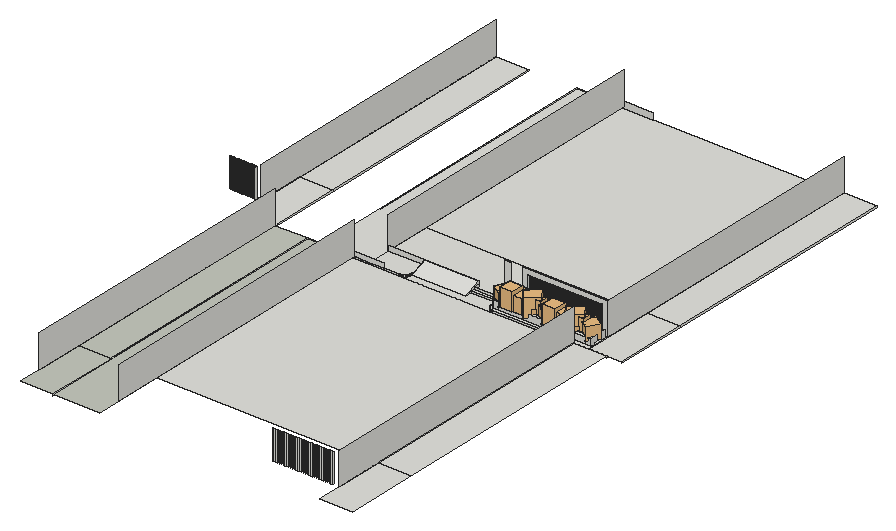
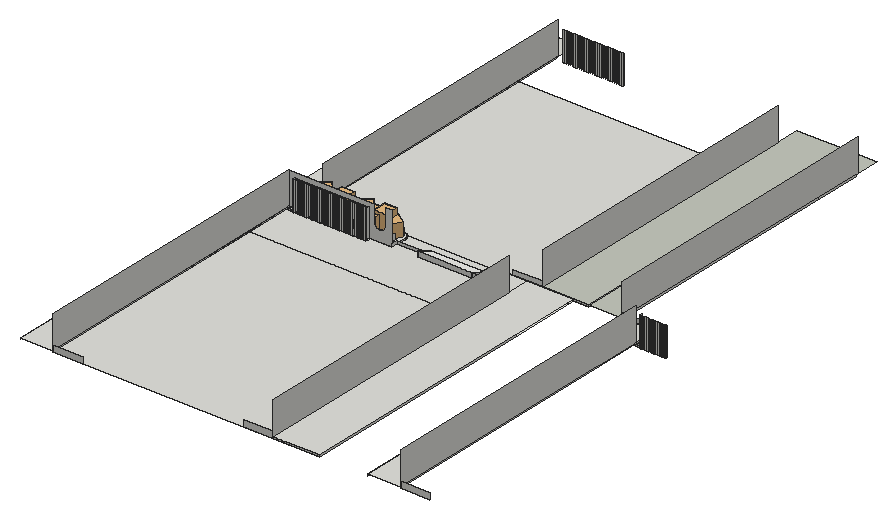
# SketchUp Ruby script. Lengths in inches.
U = 1.inch
M = Sketchup.active_model
def pt(a) = Geom::Point3d.new(a.map { |v| v * U })
def face(e, loops, mat)
  f = e.add_face(loops[0].map { |a| pt(a) })
  loops[1..].each { |l| e.add_face(l.map { |a| pt(a) }).erase! }
  f.material = f.back_material = mat if mat
  f
end
# faces: each face lists its corners as indices into pts; further lists are holes
def faces(e, pts, list, mat = nil) = list.each { |f| face(e, (f[0].is_a?(Array) ? f : [f]).map { |l| l.map { |i| pts[i] } }, mat) }
# xy, xz, yz: faces in a plane at the given z, y or x. An outline is a flat list of corners, or four numbers for a rectangle; further outlines are holes
def ring(l) = l.size == 4 ? [[l[0], l[1]], [l[2], l[1]], [l[2], l[3]], [l[0], l[3]]] : l.each_slice(2).to_a
def flat(e, list, mat, &to3) = list.each { |f| face(e, (f[0].is_a?(Array) ? f : [f]).map { |l| ring(l).map { |u, v| to3.(u, v) } }, mat) }
def xy(e, z, list, mat = nil) = flat(e, list, mat) { |x, y| [x, y, z] }
def xz(e, y, list, mat = nil) = flat(e, list, mat) { |x, z| [x, y, z] }
def yz(e, x, list, mat = nil) = flat(e, list, mat) { |y, z| [x, y, z] }
def lines(e, pts, list) = list.each { |a, b| e.add_line(pt(pts[a]), pt(pts[b])) }
# prism: a flat outline (further loops are holes) pulled along v
def prism(e, loops, v, mat = nil)
  f = face(e, loops, mat); d = Geom::Vector3d.new(v.map { |x| x * U })
  f.pushpull(f.normal.samedirection?(d) ? d.length : -d.length)
end
def box(e, o, s, mat = nil) = prism(e, [[o, [o[0] + s[0], o[1], o[2]], [o[0] + s[0], o[1] + s[1], o[2]], [o[0], o[1] + s[1], o[2]]]], [0, 0, s[2]], mat)
def at(x, y, z, deg = 0) = Geom::Transformation.translation(pt([x, y, z])) * Geom::Transformation.rotation(ORIGIN, Z_AXIS, deg.degrees)
def axes(o, x, y, z) = Geom::Transformation.new([*x, 0, *y, 0, *z, 0, *pt(o).to_a, 1])
def part(name) = M.definitions.add(name)
# library, detail: a bought-in or finely detailed component or shape, given as its bounding box
def library(name, o, s) = part(name).tap { |d| box(d.entities, o, s) }
def detail(e, o, s) = box(e.add_group.entities, o, s)
def put(e, d, t, mat = nil) = e.add_instance(d, t).tap { |i| i.material = mat if mat }
def group(e, t, mat = nil) = e.add_group.tap { |g| g.transformation = t; g.material = mat if mat }.entities
root = M.entities
M.materials.add("Material__1").color = [95, 70, 46]
M.materials.add("[0041_Chocolate]").color = [210, 105, 30]
M.materials.add("[Pavers with Grass Herringbone]").color = [197, 201, 190]
c1 = library("Areca palm plant",[0,0,0],[49.1,36.6,54.46])
c2 = library("Group\#74",[-84.69,-90.07,-0.36],[176.51,175.13,171.4])
c3 = library("Group20\#1",[-20.81,-17.08,3.79],[39.86,39.43,37.51])
c4 = library("Group38\#2",[14.01,28.44,-23.43],[18.58,18.32,38.89])
c5 = library("Group\#130",[-7.34,-1.2,0],[38.67,35.81,49.04])
c6 = part("Group\#8")
put(c6.entities,c1,axes([-6.2,56.6,6.08],[0.45017,-0.56191,0],[0.66137,0.52986,0],[0,0,0.72]))
put(c6.entities,c1,axes([-6.2,158.41,6.08],[0.45017,-0.56191,0],[0.66137,0.52986,0],[0,0,0.72]))
put(c6.entities,c2,axes([14.93,145.87,6.05],[-0.04961,-0.08593,0],[0.08593,-0.04961,0],[0,0,0.10522]))
put(c6.entities,c2,axes([14.93,193.18,6.05],[-0.04961,-0.08593,0],[0.08593,-0.04961,0],[0,0,0.10522]))
put(c6.entities,c3,axes([18.97,79.98,4.77],[0,0.85,0],[-0.85,0,0],[0,0,0.85]))
put(c6.entities,c2,axes([14.93,173.12,6.05],[-0.04961,-0.08593,0],[0.08593,-0.04961,0],[0,0,0.10522]))
g1 = group(c6.entities,at(0,0,0))
xy(g1,0,[[0,0,6,234.8],[30,0,36,234.8]])
xy(g1,3,[[6,0,30,234.8]])
xy(g1,7,[[6,5,30,229.8]],"Material__1")
xy(g1,15,[[[0,0,36,234.8],[6,5,30,229.8]]])
xz(g1,0,[[0,0,6,0,6,3,30,3,30,0,36,0,36,15,0,15]])
xz(g1,5,[[6,7,30,15]])
xz(g1,229.8,[[6,7,30,15]])
xz(g1,234.8,[[0,0,0,15,36,15,36,0,30,0,30,3,6,3,6,0]])
yz(g1,0,[[0,0,234.8,15]])
yz(g1,6,[[0,0,234.8,3],[5,7,229.8,15]])
yz(g1,30,[[0,0,234.8,3],[5,7,229.8,15]])
yz(g1,36,[[0,0,234.8,15]])
put(c6.entities,c2,axes([17.19,223.04,6.07],[-0.08133,-0.14087,0],[0.14087,-0.08133,0],[0,0,0.1725]))
put(c6.entities,c4,axes([-4.1,-1.15,28.17],[0.8848,0,0],[0,0.94674,0],[0,0,0.85826]))
put(c6.entities,c2,axes([17.19,15.79,6.07],[-0.08133,-0.14087,0],[0.14087,-0.08133,0],[0,0,0.1725]))
put(c6.entities,c2,axes([14.93,91.37,6.05],[-0.04961,-0.08593,0],[0.08593,-0.04961,0],[0,0,0.10522]))
put(c6.entities,c3,axes([18.97,181.79,4.77],[0,0.85,0],[-0.85,0,0],[0,0,0.85]))
put(c6.entities,c2,axes([14.93,44.05,6.05],[-0.04961,-0.08593,0],[0.08593,-0.04961,0],[0,0,0.10522]))
put(c6.entities,c5,axes([24.9375,191.72,8],[0,0.79,0],[-0.79,0,0],[0,0,0.79]))
put(c6.entities,c2,axes([17.19,121.23,6.07],[-0.08133,-0.14087,0],[0.14087,-0.08133,0],[0,0,0.1725]))
put(c6.entities,c4,axes([-4.1,100.66,28.17],[0.8848,0,0],[0,0.94674,0],[0,0,0.85826]))
put(c6.entities,c5,axes([24.9375,89.91,8],[0,0.79,0],[-0.79,0,0],[0,0,0.79]))
put(c6.entities,c2,axes([14.93,71.3,6.05],[-0.04961,-0.08593,0],[0.08593,-0.04961,0],[0,0,0.10522]))
xy(root,-8,[[1785.21,305.58,2364.02,838.14],[1817.65,838.14,1918.83,853.41],[1918.83,838.14,1983.13,838.14,1985.12,838.27,1987.08,838.66,1988.97,839.31,1990.76,840.19,1992.42,841.3,1993.93,842.62,1995.24,844.12,1996.35,845.78,1997.23,847.57,1997.875,849.46,1998.27,851.42,1998.4,853.41,1918.83,853.41],[1983.13,838.14,2187.9375,838.14,2185.97,838.27,2184.03,838.66,2182.17,839.29,2180.4,840.16,2178.76,841.26,2177.27,842.5625,2175.97,844.04,2174.875,845.68,2174,847.45,2173.37,849.32,2172.98,851.26,2172.86,853.22,2172.86,868.96,2115.83,868.96,2115.83,853.41,1998.4,853.41,1998.27,851.42,1997.875,849.46,1997.23,847.57,1996.35,845.78,1995.24,844.12,1993.93,842.62,1992.42,841.3,1990.76,840.19,1988.97,839.31,1987.08,838.66,1985.12,838.27],[2187.9375,838.14,2221.9375,838.14,2221.9375,853.22,2172.86,853.22,2172.98,851.26,2173.37,849.32,2174,847.45,2174.875,845.68,2175.97,844.04,2177.27,842.5625,2178.76,841.26,2180.4,840.16,2182.17,839.29,2184.03,838.66,2185.97,838.27],
  [2221.9375,838.14,2396.46,853.22],[2172.86,853.22,2221.9375,853.22,2221.9375,894.77,2223.5625,894.77,2223.5625,895.77,2224.3125,895.77,2224.3125,894.77,2227.5625,894.77,2227.5625,895.77,2228.3125,895.77,2228.3125,894.77,2231.5625,894.77,2231.5625,895.77,2232.3125,895.77,2232.3125,894.77,2235.5625,894.77,2235.5625,895.77,2236.3125,895.77,2236.3125,894.77,2239.5625,894.77,2239.5625,895.77,2240.3125,895.77,2240.3125,894.77,2243.5625,894.77,2243.5625,895.77,2244.3125,895.77,2244.3125,894.77,2247.5625,894.77,2247.5625,895.77,2248.3125,895.77,2248.3125,894.77,2251.5625,894.77,2251.5625,895.77,2252.3125,895.77,2252.3125,894.77,2255.5625,894.77,2255.5625,895.77,2256.3125,895.77,2256.3125,894.77,2259.5625,894.77,2259.5625,895.77,2260.3125,895.77,2260.3125,894.77,2263.5625,894.77,2263.5625,895.77,2264.3125,895.77,2264.3125,894.77,2267.5625,894.77,2267.5625,895.77,2268.3125,895.77,2268.3125,894.77,2271.5625,894.77,2271.5625,895.77,2272.3125,895.77,2272.3125,894.77,2275.5625,894.77,2275.5625,895.77,2276.3125,895.77,2276.3125,894.77,2279.5625,894.77,2279.5625,895.77,2280.3125,895.77,2280.3125,894.77,2283.5625,894.77,2283.5625,895.77,2284.3125,895.77,2284.3125,894.77,2287.5625,894.77,2287.5625,895.77,2288.3125,895.77,2288.3125,894.77,2291.5625,894.77,2291.5625,895.77,2292.3125,895.77,2292.3125,894.77,2295.5625,894.77,2295.5625,895.77,2296.3125,895.77,2296.3125,894.77,2299.5625,894.77,2299.5625,895.77,2300.3125,895.77,2300.3125,894.77,2303.5625,894.77,2303.5625,895.77,2304.3125,895.77,2304.3125,894.77,2307.5625,894.77,2307.5625,895.77,2308.3125,895.77,2308.3125,894.77,2311.5625,894.77,2311.5625,895.77,2312.3125,895.77,2312.3125,894.77,2315.5625,894.77,2315.5625,895.77,2316.3125,895.77,2316.3125,894.77,2319.5625,894.77,2319.5625,895.77,2320.3125,895.77,2320.3125,894.77,2323.5625,894.77,2323.5625,895.77,2324.3125,895.77,2324.3125,894.77,2327.5625,894.77,2327.5625,895.77,2328.3125,895.77,2328.3125,894.77,2331.5625,894.77,2331.5625,895.77,2332.3125,895.77,2332.3125,894.77,2335.5625,894.77,2335.5625,895.77,2336.3125,895.77,2336.3125,894.77,2339.5625,894.77,2339.5625,895.77,2340.3125,895.77,2340.3125,894.77,2343.5625,894.77,2343.5625,895.77,2344.3125,895.77,2344.3125,894.77,2347.5625,894.77,2347.5625,895.77,2348.3125,895.77,2348.3125,894.77,2351.5625,894.77,2351.5625,895.77,2352.3125,895.77,2352.3125,894.77,2355.5625,894.77,2355.5625,895.77,2356.3125,895.77,2356.3125,894.77,2359.5625,894.77,2359.5625,895.77,2360.3125,895.77,2360.3125,894.77,2363.5625,894.77,2363.5625,895.77,2364.3125,895.77,2364.3125,894.77,2367.5625,894.77,2367.5625,895.77,2368.3125,895.77,2368.3125,894.77,2371.5625,894.77,2371.5625,895.77,2372.3125,895.77,2372.3125,894.77,2375.5625,894.77,2375.5625,895.77,2376.3125,895.77,2376.3125,894.77,2379.5625,894.77,2379.5625,895.77,2380.3125,895.77,2380.3125,894.77,2396.46,894.77,2396.46,996.48,1817.65,996.48,1817.65,853.41,2115.83,853.41,2115.83,868.96,2172.86,868.96],[2221.9375,853.22,2221.9375,894.77,2383.5625,894.77,2383.5625,889.52,2396.46,889.52,2396.46,853.22],[1628.9375,889.52,1641.83,894.77],[2383.5625,889.52,2396.46,894.77],
  [1817.65,996.48,2396.46,1529.04]])
xy(root,-4.67,[[2364.02,147.25,2435.71,305.58],[2364.02,305.58,2435.71,838.14],[1641.83,838.14,1713.52,996.48],[1817.65,838.14,1918.83,1529.04],[1918.83,838.14,1983.13,838.14,1985.12,838.27,1987.08,838.66,1988.97,839.31,1990.76,840.19,1992.42,841.3,1993.93,842.62,1995.24,844.12,1996.35,845.78,1997.23,847.57,1997.875,849.46,1998.27,851.42,1998.4,853.41,1998.4,889.52,1918.83,889.52],
  [2187.9375,838.14,2396.46,838.14,2396.46,889.52,2172.86,889.52,2172.86,853.22,2172.98,851.26,2173.37,849.32,2174,847.45,2174.875,845.68,2175.97,844.04,2177.27,842.5625,2178.76,841.26,2180.4,840.16,2182.17,839.29,2184.03,838.66,2185.97,838.27],[2396.46,838.14,2468.15,996.48],[2115.83,868.96,2172.86,876.83],[2221.9375,889.52,2396.46,894.77],[1641.83,996.48,1713.52,1529.04],
  [2396.46,996.48,2468.15,1529.04]])
xy(root,-4.67,[[1713.52,147.25,1785.21,305.58],[1785.21,147.25,1886.4,838.14],[1713.52,305.58,1785.21,838.14]],"[Pavers with Grass Herringbone]")
xz(root,204.875,[[2215.125,-8,2215.875,55.1875],[2219.125,-8,2219.875,55.1875],[2223.125,-8,2223.875,55.1875],[2227.125,-8,2227.875,55.1875],[2231.125,-8,2231.875,55.1875],
  [2235.125,-8,2235.875,55.1875],[2239.125,-8,2239.875,55.1875],[2243.125,-8,2243.875,55.1875],[2247.125,-8,2247.875,55.1875],[2251.125,-8,2251.875,55.1875],
  [2255.125,-8,2255.875,55.1875],[2259.125,-8,2259.875,55.1875],[2263.125,-8,2263.875,55.1875],[2267.125,-8,2267.875,55.1875],[2271.125,-8,2271.875,55.1875],
  [2275.125,-8,2275.875,55.1875],[2279.125,-8,2279.875,55.1875],[2283.125,-8,2283.875,55.1875],[2287.125,-8,2287.875,55.1875],[2291.125,-8,2291.875,55.1875],
  [2295.125,-8,2295.875,55.1875],[2299.125,-8,2299.875,55.1875],[2303.125,-8,2303.875,55.1875],[2307.125,-8,2307.875,55.1875],[2311.125,-8,2311.875,55.1875],
  [2315.125,-8,2315.875,55.1875],[2319.125,-8,2319.875,55.1875],[2323.125,-8,2323.875,55.1875],[2327.125,-8,2327.875,55.1875],[2331.125,-8,2331.875,55.1875],
  [2335.125,-8,2335.875,55.1875],[2339.125,-8,2339.875,55.1875],[2343.125,-8,2343.875,55.1875],[2347.125,-8,2347.875,55.1875]])
xz(root,838.14,[[1641.83,-8,1650.02,-4.67],[1650.02,-8,1713.52,-4.67],[1785.21,-8,1817.65,-4.67],[1817.65,-8,1889.33,-4.67],[1889.33,-8,1918.83,-4.67],
  [1918.83,-8,1949.9,-4.67],[1949.9,-8,1983.13,-4.67],[2187.9375,-8,2221.9375,-4.67],[2221.9375,-8,2300.52,-4.67],[2300.52,-8,2364.02,-4.67],
  [2364.02,-8,2396.46,-4.67],[2396.46,-8,2435.71,-4.67],[1650.02,-4.67,1713.52,6.125],[1886.4,-4.67,1949.9,6.125],[2300.52,-4.67,2364.02,6.125]])
xz(root,868.96,[[2115.83,-8,2172.86,-4.67]])
xz(root,876.83,[[2115.83,-4.67,2172.86,0.73]])
xz(root,889.52,[[1628.9375,-8,1641.83,-4.67],[2383.5625,-8,2396.46,-4.67],[1918.83,-4.67,1998.4,6.125],[1998.4,-4.67,2115.83,6.125],[2172.86,-4.67,2221.9375,-4.67,2221.9375,55.1875,2383.5625,55.1875,2383.5625,-4.67,2396.46,-4.67,2396.46,66.125,2210.54,66.125,2210.54,26.79,2209.65,24.11,2208.18,21.71,2206.21,19.69,2203.84,18.17,2201.18,17.23,2198.38,16.91,2195.58,17.23,2192.92,18.17,2190.55,19.69,2188.58,21.71,2187.11,24.11,2186.22,26.79,2186.22,66.125,2173.1,66.125,2173.1,6.125,2172.86,6.125]])
xz(root,894.77,[[1569.6875,-8,1572.9375,-4.67],[1572.9375,-8,1573.6875,-4.67],[1573.6875,-8,1576.9375,-4.67],[1576.9375,-8,1577.6875,-4.67],[1577.6875,-8,1580.9375,-4.67],
  [1580.9375,-8,1581.6875,-4.67],[1581.6875,-8,1584.9375,-4.67],[1584.9375,-8,1585.6875,-4.67],[1585.6875,-8,1588.9375,-4.67],[1588.9375,-8,1589.6875,-4.67],
  [1589.6875,-8,1592.9375,-4.67],[1592.9375,-8,1593.6875,-4.67],[1593.6875,-8,1596.9375,-4.67],[1596.9375,-8,1597.6875,-4.67],[1597.6875,-8,1600.9375,-4.67],
  [1600.9375,-8,1601.6875,-4.67],[1601.6875,-8,1604.9375,-4.67],[1604.9375,-8,1605.6875,-4.67],[1605.6875,-8,1608.9375,-4.67],[1608.9375,-8,1609.6875,-4.67],
  [1609.6875,-8,1612.9375,-4.67],[1612.9375,-8,1613.6875,-4.67],[1613.6875,-8,1616.9375,-4.67],[1616.9375,-8,1617.6875,-4.67],[1617.6875,-8,1620.9375,-4.67],
  [1620.9375,-8,1621.6875,-4.67],[1621.6875,-8,1624.9375,-4.67],[1624.9375,-8,1625.6875,-4.67],[1625.6875,-8,1628.9375,-4.67],[1628.9375,-8,1641.83,-4.67],
  [2221.9375,-8,2223.5625,-4.67],[2223.5625,-8,2224.3125,-4.67],[2224.3125,-8,2227.5625,-4.67],[2227.5625,-8,2228.3125,-4.67],[2228.3125,-8,2231.5625,-4.67],
  [2231.5625,-8,2232.3125,-4.67],[2232.3125,-8,2235.5625,-4.67],[2235.5625,-8,2236.3125,-4.67],[2236.3125,-8,2239.5625,-4.67],[2239.5625,-8,2240.3125,-4.67],
  [2240.3125,-8,2243.5625,-4.67],[2243.5625,-8,2244.3125,-4.67],[2244.3125,-8,2247.5625,-4.67],[2247.5625,-8,2248.3125,-4.67],[2248.3125,-8,2251.5625,-4.67],
  [2251.5625,-8,2252.3125,-4.67],[2252.3125,-8,2255.5625,-4.67],[2255.5625,-8,2256.3125,-4.67],[2256.3125,-8,2259.5625,-4.67],[2259.5625,-8,2260.3125,-4.67],
  [2260.3125,-8,2263.5625,-4.67],[2263.5625,-8,2264.3125,-4.67],[2264.3125,-8,2267.5625,-4.67],[2267.5625,-8,2268.3125,-4.67],[2268.3125,-8,2271.5625,-4.67],
  [2271.5625,-8,2272.3125,-4.67],[2272.3125,-8,2275.5625,-4.67],[2275.5625,-8,2276.3125,-4.67],[2276.3125,-8,2279.5625,-4.67],[2279.5625,-8,2280.3125,-4.67],
  [2280.3125,-8,2283.5625,-4.67],[2283.5625,-8,2284.3125,-4.67],[2284.3125,-8,2287.5625,-4.67],[2287.5625,-8,2288.3125,-4.67],[2288.3125,-8,2291.5625,-4.67],
  [2291.5625,-8,2292.3125,-4.67],[2292.3125,-8,2295.5625,-4.67],[2295.5625,-8,2296.3125,-4.67],[2296.3125,-8,2299.5625,-4.67],[2299.5625,-8,2300.3125,-4.67],
  [2300.3125,-8,2303.5625,-4.67],[2303.5625,-8,2304.3125,-4.67],[2304.3125,-8,2307.5625,-4.67],[2307.5625,-8,2308.3125,-4.67],[2308.3125,-8,2311.5625,-4.67],
  [2311.5625,-8,2312.3125,-4.67],[2312.3125,-8,2315.5625,-4.67],[2315.5625,-8,2316.3125,-4.67],[2316.3125,-8,2319.5625,-4.67],[2319.5625,-8,2320.3125,-4.67],
  [2320.3125,-8,2323.5625,-4.67],[2323.5625,-8,2324.3125,-4.67],[2324.3125,-8,2327.5625,-4.67],[2327.5625,-8,2328.3125,-4.67],[2328.3125,-8,2331.5625,-4.67],
  [2331.5625,-8,2332.3125,-4.67],[2332.3125,-8,2335.5625,-4.67],[2335.5625,-8,2336.3125,-4.67],[2336.3125,-8,2339.5625,-4.67],[2339.5625,-8,2340.3125,-4.67],
  [2340.3125,-8,2343.5625,-4.67],[2343.5625,-8,2344.3125,-4.67],[2344.3125,-8,2347.5625,-4.67],[2347.5625,-8,2348.3125,-4.67],[2348.3125,-8,2351.5625,-4.67],
  [2351.5625,-8,2352.3125,-4.67],[2352.3125,-8,2355.5625,-4.67],[2355.5625,-8,2356.3125,-4.67],[2356.3125,-8,2359.5625,-4.67],[2359.5625,-8,2360.3125,-4.67],
  [2360.3125,-8,2363.5625,-4.67],[2363.5625,-8,2364.3125,-4.67],[2364.3125,-8,2367.5625,-4.67],[2367.5625,-8,2368.3125,-4.67],[2368.3125,-8,2371.5625,-4.67],
  [2371.5625,-8,2372.3125,-4.67],[2372.3125,-8,2375.5625,-4.67],[2375.5625,-8,2376.3125,-4.67],[2376.3125,-8,2379.5625,-4.67],[2379.5625,-8,2380.3125,-4.67],
  [2380.3125,-8,2383.5625,-4.67],[2383.5625,-8,2396.46,-4.67]])
xz(root,894.77,[[1569.6875,-4.67,1572.9375,55.1875],[1573.6875,-4.67,1576.9375,55.1875],[1577.6875,-4.67,1580.9375,55.1875],[1581.6875,-4.67,1584.9375,55.1875],[1585.6875,-4.67,1588.9375,55.1875],
  [1589.6875,-4.67,1592.9375,55.1875],[1593.6875,-4.67,1596.9375,55.1875],[1597.6875,-4.67,1600.9375,55.1875],[1601.6875,-4.67,1604.9375,55.1875],[1605.6875,-4.67,1608.9375,55.1875],
  [1609.6875,-4.67,1612.9375,55.1875],[1613.6875,-4.67,1616.9375,55.1875],[1617.6875,-4.67,1620.9375,55.1875],[1621.6875,-4.67,1624.9375,55.1875],[1625.6875,-4.67,1628.9375,55.1875],
  [2221.9375,-4.67,2223.5625,55.1875],[2224.3125,-4.67,2227.5625,55.1875],[2228.3125,-4.67,2231.5625,55.1875],[2232.3125,-4.67,2235.5625,55.1875],[2236.3125,-4.67,2239.5625,55.1875],
  [2240.3125,-4.67,2243.5625,55.1875],[2244.3125,-4.67,2247.5625,55.1875],[2248.3125,-4.67,2251.5625,55.1875],[2252.3125,-4.67,2255.5625,55.1875],[2256.3125,-4.67,2259.5625,55.1875],
  [2260.3125,-4.67,2263.5625,55.1875],[2264.3125,-4.67,2267.5625,55.1875],[2268.3125,-4.67,2271.5625,55.1875],[2272.3125,-4.67,2275.5625,55.1875],[2276.3125,-4.67,2279.5625,55.1875],
  [2280.3125,-4.67,2283.5625,55.1875],[2284.3125,-4.67,2287.5625,55.1875],[2288.3125,-4.67,2291.5625,55.1875],[2292.3125,-4.67,2295.5625,55.1875],[2296.3125,-4.67,2299.5625,55.1875],
  [2300.3125,-4.67,2303.5625,55.1875],[2304.3125,-4.67,2307.5625,55.1875],[2308.3125,-4.67,2311.5625,55.1875],[2312.3125,-4.67,2315.5625,55.1875],[2316.3125,-4.67,2319.5625,55.1875],
  [2320.3125,-4.67,2323.5625,55.1875],[2324.3125,-4.67,2327.5625,55.1875],[2328.3125,-4.67,2331.5625,55.1875],[2332.3125,-4.67,2335.5625,55.1875],[2336.3125,-4.67,2339.5625,55.1875],
  [2340.3125,-4.67,2343.5625,55.1875],[2344.3125,-4.67,2347.5625,55.1875],[2348.3125,-4.67,2351.5625,55.1875],[2352.3125,-4.67,2355.5625,55.1875],[2356.3125,-4.67,2359.5625,55.1875],
  [2360.3125,-4.67,2363.5625,55.1875],[2364.3125,-4.67,2367.5625,55.1875],[2368.3125,-4.67,2371.5625,55.1875],[2372.3125,-4.67,2375.5625,55.1875],[2376.3125,-4.67,2379.5625,55.1875],
  [2380.3125,-4.67,2383.5625,55.1875]],"[0041_Chocolate]")
xz(root,895.77,[[1572.9375,-8,1573.6875,55.1875],[1576.9375,-8,1577.6875,55.1875],[1580.9375,-8,1581.6875,55.1875],[1584.9375,-8,1585.6875,55.1875],[1588.9375,-8,1589.6875,55.1875],
  [1592.9375,-8,1593.6875,55.1875],[1596.9375,-8,1597.6875,55.1875],[1600.9375,-8,1601.6875,55.1875],[1604.9375,-8,1605.6875,55.1875],[1608.9375,-8,1609.6875,55.1875],
  [1612.9375,-8,1613.6875,55.1875],[1616.9375,-8,1617.6875,55.1875],[1620.9375,-8,1621.6875,55.1875],[1624.9375,-8,1625.6875,55.1875],[2223.5625,-8,2224.3125,55.1875],
  [2227.5625,-8,2228.3125,55.1875],[2231.5625,-8,2232.3125,55.1875],[2235.5625,-8,2236.3125,55.1875],[2239.5625,-8,2240.3125,55.1875],[2243.5625,-8,2244.3125,55.1875],
  [2247.5625,-8,2248.3125,55.1875],[2251.5625,-8,2252.3125,55.1875],[2255.5625,-8,2256.3125,55.1875],[2259.5625,-8,2260.3125,55.1875],[2263.5625,-8,2264.3125,55.1875],
  [2267.5625,-8,2268.3125,55.1875],[2271.5625,-8,2272.3125,55.1875],[2275.5625,-8,2276.3125,55.1875],[2279.5625,-8,2280.3125,55.1875],[2283.5625,-8,2284.3125,55.1875],
  [2287.5625,-8,2288.3125,55.1875],[2291.5625,-8,2292.3125,55.1875],[2295.5625,-8,2296.3125,55.1875],[2299.5625,-8,2300.3125,55.1875],[2303.5625,-8,2304.3125,55.1875],
  [2307.5625,-8,2308.3125,55.1875],[2311.5625,-8,2312.3125,55.1875],[2315.5625,-8,2316.3125,55.1875],[2319.5625,-8,2320.3125,55.1875],[2323.5625,-8,2324.3125,55.1875],
  [2327.5625,-8,2328.3125,55.1875],[2331.5625,-8,2332.3125,55.1875],[2335.5625,-8,2336.3125,55.1875],[2339.5625,-8,2340.3125,55.1875],[2343.5625,-8,2344.3125,55.1875],
  [2347.5625,-8,2348.3125,55.1875],[2351.5625,-8,2352.3125,55.1875],[2355.5625,-8,2356.3125,55.1875],[2359.5625,-8,2360.3125,55.1875],[2363.5625,-8,2364.3125,55.1875],
  [2367.5625,-8,2368.3125,55.1875],[2371.5625,-8,2372.3125,55.1875],[2375.5625,-8,2376.3125,55.1875],[2379.5625,-8,2380.3125,55.1875]])
xz(root,1529.04,[[1578.33,-8,1641.83,6.125],[1817.65,-8,1817.65,-4.67,1918.83,-4.67,1918.83,6.125,1982.33,6.125,1982.33,-8],[2332.96,-8,2396.46,6.125]])
yz(root,1572.9375,[[894.77,-8,895.77,55.1875]])
yz(root,1573.6875,[[894.77,-8,895.77,55.1875]])
yz(root,1576.9375,[[894.77,-8,895.77,55.1875]])
yz(root,1577.6875,[[894.77,-8,895.77,55.1875]])
yz(root,1580.9375,[[894.77,-8,895.77,55.1875]])
yz(root,1581.6875,[[894.77,-8,895.77,55.1875]])
yz(root,1584.9375,[[894.77,-8,895.77,55.1875]])
yz(root,1585.6875,[[894.77,-8,895.77,55.1875]])
yz(root,1588.9375,[[894.77,-8,895.77,55.1875]])
yz(root,1589.6875,[[894.77,-8,895.77,55.1875]])
yz(root,1592.9375,[[894.77,-8,895.77,55.1875]])
yz(root,1593.6875,[[894.77,-8,895.77,55.1875]])
yz(root,1596.9375,[[894.77,-8,895.77,55.1875]])
yz(root,1597.6875,[[894.77,-8,895.77,55.1875]])
yz(root,1600.9375,[[894.77,-8,895.77,55.1875]])
yz(root,1601.6875,[[894.77,-8,895.77,55.1875]])
yz(root,1604.9375,[[894.77,-8,895.77,55.1875]])
yz(root,1605.6875,[[894.77,-8,895.77,55.1875]])
yz(root,1608.9375,[[894.77,-8,895.77,55.1875]])
yz(root,1609.6875,[[894.77,-8,895.77,55.1875]])
yz(root,1612.9375,[[894.77,-8,895.77,55.1875]])
yz(root,1613.6875,[[894.77,-8,895.77,55.1875]])
yz(root,1616.9375,[[894.77,-8,895.77,55.1875]])
yz(root,1617.6875,[[894.77,-8,895.77,55.1875]])
yz(root,1620.9375,[[894.77,-8,895.77,55.1875]])
yz(root,1621.6875,[[894.77,-8,895.77,55.1875]])
yz(root,1624.9375,[[894.77,-8,895.77,55.1875]])
yz(root,1625.6875,[[894.77,-8,895.77,55.1875]])
yz(root,1628.9375,[[889.52,-8,894.77,55.1875]])
yz(root,1641.83,[[838.14,-8,889.52,-4.67],[889.52,-8,894.77,-4.67],[894.77,-8,996.48,-4.67],[996.48,-8,1529.04,-4.67],[889.52,-4.67,1529.04,66.125]])
yz(root,1713.52,[[203.875,-8,305.58,-4.67],[305.58,-8,838.14,-4.67],[838.14,-8,996.48,-4.67],[996.48,-8,1529.04,-4.67],[198.625,-4.67,838.14,66.125]])
yz(root,1785.21,[[147.25,-8,305.58,-4.67],[305.58,-8,838.14,-4.67]])
yz(root,1817.65,[[996.48,-8,1529.04,-4.67]])
yz(root,1886.4,[[198.625,-4.67,838.14,66.125]])
yz(root,1918.83,[[889.52,-4.67,1529.04,66.125]])
yz(root,1998.4,[[853.41,-8,861.93,-4.67,853.41,-4.67],[861.93,-4.67,889.52,6.125,889.52,-4.67]])
yz(root,2115.83,[[853.41,-8,868.96,-8,868.96,-4.67,861.93,-4.67],[861.93,-4.67,876.83,-4.67,876.83,0.73,889.52,0.73,889.52,6.125],[876.83,-4.67,889.52,0.73]])
yz(root,2172.86,[[853.22,-8,868.96,-4.67],[876.83,-4.67,889.52,0.73]])
yz(root,2221.9375,[[889.52,-4.67,894.77,55.1875]])
yz(root,2223.5625,[[894.77,-8,895.77,55.1875]])
yz(root,2224.3125,[[894.77,-8,895.77,55.1875]])
yz(root,2227.5625,[[894.77,-8,895.77,55.1875]])
yz(root,2228.3125,[[894.77,-8,895.77,55.1875]])
yz(root,2231.5625,[[894.77,-8,895.77,55.1875]])
yz(root,2232.3125,[[894.77,-8,895.77,55.1875]])
yz(root,2235.5625,[[894.77,-8,895.77,55.1875]])
yz(root,2236.3125,[[894.77,-8,895.77,55.1875]])
yz(root,2239.5625,[[894.77,-8,895.77,55.1875]])
yz(root,2240.3125,[[894.77,-8,895.77,55.1875]])
yz(root,2243.5625,[[894.77,-8,895.77,55.1875]])
yz(root,2244.3125,[[894.77,-8,895.77,55.1875]])
yz(root,2247.5625,[[894.77,-8,895.77,55.1875]])
yz(root,2248.3125,[[894.77,-8,895.77,55.1875]])
yz(root,2251.5625,[[894.77,-8,895.77,55.1875]])
yz(root,2252.3125,[[894.77,-8,895.77,55.1875]])
yz(root,2255.5625,[[894.77,-8,895.77,55.1875]])
yz(root,2256.3125,[[894.77,-8,895.77,55.1875]])
yz(root,2259.5625,[[894.77,-8,895.77,55.1875]])
yz(root,2260.3125,[[894.77,-8,895.77,55.1875]])
yz(root,2263.5625,[[894.77,-8,895.77,55.1875]])
yz(root,2264.3125,[[894.77,-8,895.77,55.1875]])
yz(root,2267.5625,[[894.77,-8,895.77,55.1875]])
yz(root,2268.3125,[[894.77,-8,895.77,55.1875]])
yz(root,2271.5625,[[894.77,-8,895.77,55.1875]])
yz(root,2272.3125,[[894.77,-8,895.77,55.1875]])
yz(root,2275.5625,[[894.77,-8,895.77,55.1875]])
yz(root,2276.3125,[[894.77,-8,895.77,55.1875]])
yz(root,2279.5625,[[894.77,-8,895.77,55.1875]])
yz(root,2280.3125,[[894.77,-8,895.77,55.1875]])
yz(root,2283.5625,[[894.77,-8,895.77,55.1875]])
yz(root,2284.3125,[[894.77,-8,895.77,55.1875]])
yz(root,2287.5625,[[894.77,-8,895.77,55.1875]])
yz(root,2288.3125,[[894.77,-8,895.77,55.1875]])
yz(root,2291.5625,[[894.77,-8,895.77,55.1875]])
yz(root,2292.3125,[[894.77,-8,895.77,55.1875]])
yz(root,2295.5625,[[894.77,-8,895.77,55.1875]])
yz(root,2296.3125,[[894.77,-8,895.77,55.1875]])
yz(root,2299.5625,[[894.77,-8,895.77,55.1875]])
yz(root,2300.3125,[[894.77,-8,895.77,55.1875]])
yz(root,2303.5625,[[894.77,-8,895.77,55.1875]])
yz(root,2304.3125,[[894.77,-8,895.77,55.1875]])
yz(root,2307.5625,[[894.77,-8,895.77,55.1875]])
yz(root,2308.3125,[[894.77,-8,895.77,55.1875]])
yz(root,2311.5625,[[894.77,-8,895.77,55.1875]])
yz(root,2312.3125,[[894.77,-8,895.77,55.1875]])
yz(root,2315.5625,[[894.77,-8,895.77,55.1875]])
yz(root,2316.3125,[[894.77,-8,895.77,55.1875]])
yz(root,2319.5625,[[894.77,-8,895.77,55.1875]])
yz(root,2320.3125,[[894.77,-8,895.77,55.1875]])
yz(root,2323.5625,[[894.77,-8,895.77,55.1875]])
yz(root,2324.3125,[[894.77,-8,895.77,55.1875]])
yz(root,2327.5625,[[894.77,-8,895.77,55.1875]])
yz(root,2328.3125,[[894.77,-8,895.77,55.1875]])
yz(root,2331.5625,[[894.77,-8,895.77,55.1875]])
yz(root,2332.3125,[[894.77,-8,895.77,55.1875]])
yz(root,2335.5625,[[894.77,-8,895.77,55.1875]])
yz(root,2336.3125,[[894.77,-8,895.77,55.1875]])
yz(root,2339.5625,[[894.77,-8,895.77,55.1875]])
yz(root,2340.3125,[[894.77,-8,895.77,55.1875]])
yz(root,2343.5625,[[894.77,-8,895.77,55.1875]])
yz(root,2344.3125,[[894.77,-8,895.77,55.1875]])
yz(root,2347.5625,[[894.77,-8,895.77,55.1875]])
yz(root,2348.3125,[[894.77,-8,895.77,55.1875]])
yz(root,2351.5625,[[894.77,-8,895.77,55.1875]])
yz(root,2352.3125,[[894.77,-8,895.77,55.1875]])
yz(root,2355.5625,[[894.77,-8,895.77,55.1875]])
yz(root,2356.3125,[[894.77,-8,895.77,55.1875]])
yz(root,2359.5625,[[894.77,-8,895.77,55.1875]])
yz(root,2360.3125,[[894.77,-8,895.77,55.1875]])
yz(root,2363.5625,[[894.77,-8,895.77,55.1875]])
yz(root,2364.02,[[203.875,-8,305.58,-4.67],[305.58,-8,838.14,-4.67],[198.625,-4.67,838.14,66.125]])
yz(root,2364.3125,[[894.77,-8,895.77,55.1875]])
yz(root,2367.5625,[[894.77,-8,895.77,55.1875]])
yz(root,2368.3125,[[894.77,-8,895.77,55.1875]])
yz(root,2371.5625,[[894.77,-8,895.77,55.1875]])
yz(root,2372.3125,[[894.77,-8,895.77,55.1875]])
yz(root,2375.5625,[[894.77,-8,895.77,55.1875]])
yz(root,2376.3125,[[894.77,-8,895.77,55.1875]])
yz(root,2379.5625,[[894.77,-8,895.77,55.1875]])
yz(root,2380.3125,[[894.77,-8,895.77,55.1875]])
yz(root,2383.5625,[[889.52,-8,894.77,55.1875]])
yz(root,2396.46,[[838.14,-8,889.52,-4.67],[889.52,-8,894.77,-4.67],[894.77,-8,996.48,-4.67],[996.48,-8,1529.04,-4.67],[889.52,-4.67,1529.04,66.125]])
yz(root,2468.15,[[838.14,-8,996.48,-4.67],[996.48,-8,1529.04,-4.67]])
p = [[1985.12,838.27,-4.67],[1983.13,838.14,-4.67],[1983.13,838.14,-8],[1985.12,838.27,-8],[2187.9375,838.14,-4.67],[2185.97,838.27,-4.67],
  [2185.97,838.27,-8],[2187.9375,838.14,-8],[1987.08,838.66,-4.67],[1987.08,838.66,-8],[2184.03,838.66,-4.67],[2184.03,838.66,-8],
  [1988.97,839.31,-4.67],[1988.97,839.31,-8],[2182.17,839.29,-4.67],[2182.17,839.29,-8],[1990.76,840.19,-4.67],[1990.76,840.19,-8],
  [2180.4,840.16,-4.67],[2180.4,840.16,-8],[1992.42,841.3,-4.67],[1992.42,841.3,-8],[2178.76,841.26,-4.67],[2178.76,841.26,-8],
  [1993.93,842.62,-4.67],[1993.93,842.62,-8],[2177.27,842.5625,-4.67],[2177.27,842.5625,-8],[1995.24,844.12,-4.67],[1995.24,844.12,-8],
  [2175.97,844.04,-4.67],[2175.97,844.04,-8],[2174.875,845.68,-4.67],[2174.875,845.68,-8],[1996.35,845.78,-4.67],[1996.35,845.78,-8],
  [2174,847.45,-4.67],[2174,847.45,-8],[1997.23,847.57,-4.67],[1997.23,847.57,-8],[2173.37,849.32,-4.67],[2173.37,849.32,-8],
  [1997.875,849.46,-4.67],[1997.875,849.46,-8],[2172.98,851.26,-4.67],[2172.98,851.26,-8],[1998.27,851.42,-4.67],[1998.27,851.42,-8],
  [2172.86,853.22,-4.67],[2172.86,853.22,-8],[1998.4,853.41,-4.67],[1998.4,853.41,-8],[2115.83,853.41,-8],[2115.83,861.93,-4.67],
  [2115.83,889.52,6.125],[1998.4,889.52,6.125],[1998.4,861.93,-4.67]]
faces(root,p,[[0,1,2,3],[4,5,6,7],[8,0,3,9],[5,10,11,6],[12,8,9,13],[10,14,15,11],[16,12,13,17],[14,18,19,15],
  [20,16,17,21],[18,22,23,19],[24,20,21,25],[22,26,27,23],[28,24,25,29],[26,30,31,27],[30,32,33,31],[34,28,29,35],
  [32,36,37,33],[38,34,35,39],[36,40,41,37],[42,38,39,43],[40,44,45,41],[46,42,43,47],[44,48,49,45],[50,46,47,51],
  [52,53,54,55,56,51]])
put(root,c6,axes([2394,847.2,-4.73],[0,1,0],[-0.9127,0,0],[0,0,1]))
